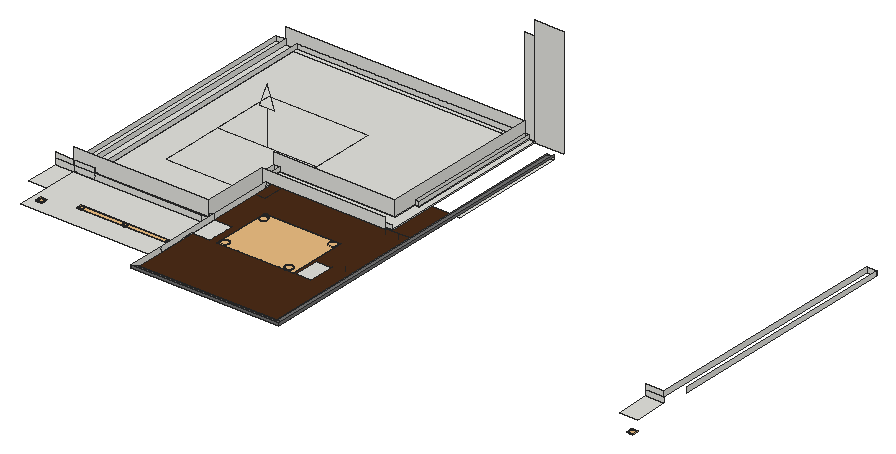
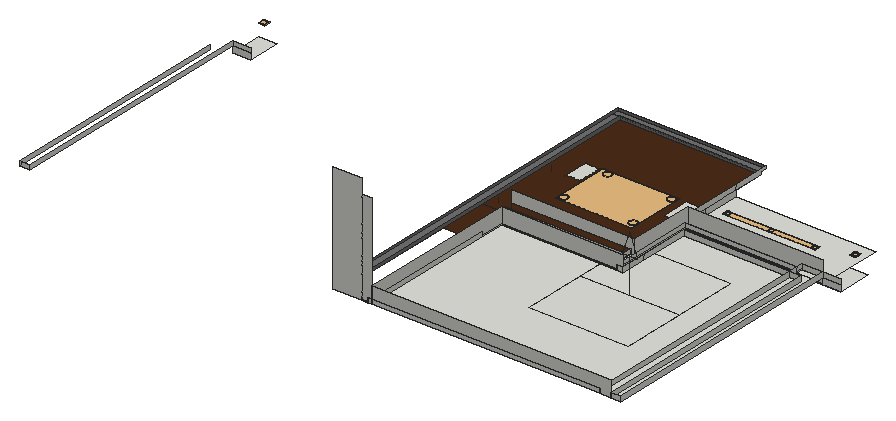
# SketchUp Ruby script. Lengths in inches.
U = 1.inch
M = Sketchup.active_model
def pt(a) = Geom::Point3d.new(a.map { |v| v * U })
def face(e, loops, mat)
  f = e.add_face(loops[0].map { |a| pt(a) })
  loops[1..].each { |l| e.add_face(l.map { |a| pt(a) }).erase! }
  f.material = f.back_material = mat if mat
  f
end
# faces: each face lists its corners as indices into pts; further lists are holes
def faces(e, pts, list, mat = nil) = list.each { |f| face(e, (f[0].is_a?(Array) ? f : [f]).map { |l| l.map { |i| pts[i] } }, mat) }
# xy, xz, yz: faces in a plane at the given z, y or x. An outline is a flat list of corners, or four numbers for a rectangle; further outlines are holes
def ring(l) = l.size == 4 ? [[l[0], l[1]], [l[2], l[1]], [l[2], l[3]], [l[0], l[3]]] : l.each_slice(2).to_a
def flat(e, list, mat, &to3) = list.each { |f| face(e, (f[0].is_a?(Array) ? f : [f]).map { |l| ring(l).map { |u, v| to3.(u, v) } }, mat) }
def xy(e, z, list, mat = nil) = flat(e, list, mat) { |x, y| [x, y, z] }
def xz(e, y, list, mat = nil) = flat(e, list, mat) { |x, z| [x, y, z] }
def yz(e, x, list, mat = nil) = flat(e, list, mat) { |y, z| [x, y, z] }
def lines(e, pts, list) = list.each { |a, b| e.add_line(pt(pts[a]), pt(pts[b])) }
# prism: a flat outline (further loops are holes) pulled along v
def prism(e, loops, v, mat = nil)
  f = face(e, loops, mat); d = Geom::Vector3d.new(v.map { |x| x * U })
  f.pushpull(f.normal.samedirection?(d) ? d.length : -d.length)
end
def box(e, o, s, mat = nil) = prism(e, [[o, [o[0] + s[0], o[1], o[2]], [o[0] + s[0], o[1] + s[1], o[2]], [o[0], o[1] + s[1], o[2]]]], [0, 0, s[2]], mat)
def at(x, y, z, deg = 0) = Geom::Transformation.translation(pt([x, y, z])) * Geom::Transformation.rotation(ORIGIN, Z_AXIS, deg.degrees)
def axes(o, x, y, z) = Geom::Transformation.new([*x, 0, *y, 0, *z, 0, *pt(o).to_a, 1])
def part(name) = M.definitions.add(name)
# library, detail: a bought-in or finely detailed component or shape, given as its bounding box
def library(name, o, s) = part(name).tap { |d| box(d.entities, o, s) }
def detail(e, o, s) = box(e.add_group.entities, o, s)
def put(e, d, t, mat = nil) = e.add_instance(d, t).tap { |i| i.material = mat if mat }
def group(e, t, mat = nil) = e.add_group.tap { |g| g.transformation = t; g.material = mat if mat }.entities
root = M.entities
M.materials.add("[Color M05]").color = [114, 114, 114]
M.materials.add("[Wood Veneer 01]").color = [76, 44, 23]
c1 = library("Group\#26",[-0.5,-0.5,-0.1],[9.125,9.125,0.2])
c2 = library("Group\#20",[-0.5,-0.5,-0.1],[139.5,7.875,0.2])
c3 = library("Group\#21",[-0.5,-0.5,-0.1],[115.36,88.99,0.2])
c4 = part("Group266\#1")
p = [[0,0,0],[0,0,-53.16],[-11.52,0,-53.16],[75.01,-97.09,0],[-75.01,-97.09,0],[75.01,97.09,0],
  [75.01,0,0],[-75.01,97.09,0],[11.52,0,-53.16],[-75.01,0,0],[0,0,-86.05]]
lines(c4.entities,p,[[0,1],[1,2],[3,4],[5,6],[7,5],[1,8],[9,0],[0,6],[8,10],[4,9],[6,3],[2,10],
  [9,7]])
c5 = part("Rectangle Light\#1")
put(c5.entities,c4,at(0,0,0))
xy(root,104.8125,[[252.74,1588.1,279.74,1638.35],[1145.33,1588.1,1172.33,1638.35]])
xy(root,104.9375,[[[279.74,1537.85,491.71,1638.35],[294.3,1555.5,295.35,1555.63,296.33,1556.04,297.18,1556.6875,297.82,1557.53,298.23,1558.51,298.37,1559.56,298.23,1560.61,297.82,1561.59,297.18,1562.43,296.33,1563.08,295.35,1563.48,294.3,1563.62,293.25,1563.48,292.27,1563.08,291.43,1562.43,290.79,1561.59,290.38,1560.61,290.24,1559.56,290.38,1558.51,290.79,1557.53,291.43,1556.6875,292.27,1556.04,293.25,1555.63],[342.36,1572.17,343.25,1572.29,344.08,1572.63,344.79,1573.18,345.34,1573.89,345.68,1574.72,345.8,1575.61,345.68,1576.5,345.34,1577.33,344.79,1578.04,344.08,1578.59,343.25,1578.93,342.36,1579.05,341.47,1578.93,340.64,1578.59,339.93,1578.04,339.38,1577.33,339.04,1576.5,338.92,1575.61,339.04,1574.72,339.38,1573.89,339.93,1573.18,340.64,1572.63,341.47,1572.29],[408.17,1572.17,409.0625,1572.29,409.89,1572.63,410.6,1573.18,411.15,1573.89,411.49,1574.72,411.61,1575.61,411.49,1576.5,411.15,1577.33,410.6,1578.04,409.89,1578.59,409.0625,1578.93,408.17,1579.05,407.28,1578.93,406.45,1578.59,405.74,1578.04,405.2,1577.33,404.85,1576.5,404.74,1575.61,404.85,1574.72,405.2,1573.89,405.74,1573.18,406.45,1572.63,407.28,1572.29],[473.99,1572.17,474.875,1572.29,475.7,1572.63,476.42,1573.18,476.96,1573.89,477.31,1574.72,477.42,1575.61,477.31,1576.5,476.96,1577.33,476.42,1578.04,475.7,1578.59,474.875,1578.93,473.99,1579.05,473.1,1578.93,472.27,1578.59,471.55,1578.04,471.01,1577.33,470.66,1576.5,470.55,1575.61,470.66,1574.72,471.01,1573.89,471.55,1573.18,472.27,1572.63,473.1,1572.29]]])
xy(root,113.8125,[[491.71,1597.35,519.14,1638.29],[649.86,1597.35,671.36,1634.91],[279.74,1638.35,312.05,1647.57],[312.05,1638.35,472.88,1647.57],[279.74,1647.57,312.05,1647.57,312.05,1661.875,294.47,1661.875,294.47,2020.66,279.74,2020.66],
  [294.47,1661.875,312.05,2020.66],[312.05,1661.875,312.05,2013.29,655.66,2013.29,655.66,1775.97,471.68,1775.97,471.68,1661.875],[662.14,1749.22,671.36,2020.66],[704.8,1824.2,715.11,2001.02],[312.05,2013.29,624.8,2020.66],
  [624.8,2013.29,655.66,2020.66]])
xy(root,113.8125,[[[491.71,1490.47,491.71,1597.35,519.14,1597.35,519.14,1638.29,491.71,1638.29,491.71,1749.22,704.8,1749.22,704.8,1490.47],[649.86,1597.35,671.36,1634.91],[633.34,1597.54,634.9,1597.75,636.34,1598.35,637.58,1599.3,638.54,1600.54,639.14,1601.99,639.34,1603.54,639.14,1605.1,638.54,1606.54,637.58,1607.79,636.34,1608.74,634.9,1609.34,633.34,1609.54,631.79,1609.34,630.34,1608.74,629.1,1607.79,628.15,1606.54,627.55,1605.1,627.34,1603.54,627.55,1601.99,628.15,1600.54,629.1,1599.3,630.34,1598.35,631.79,1597.75],[536.53,1597.54,538.08,1597.75,539.53,1598.35,540.77,1599.3,541.73,1600.54,542.33,1601.99,542.53,1603.54,542.33,1605.1,541.73,1606.54,540.77,1607.79,539.53,1608.74,538.08,1609.34,536.53,1609.54,534.98,1609.34,533.53,1608.74,532.29,1607.79,531.33,1606.54,530.73,1605.1,530.53,1603.54,530.73,1601.99,531.33,1600.54,532.29,1599.3,533.53,1598.35,534.98,1597.75],[536.53,1670.29,538.08,1670.5,539.53,1671.1,540.77,1672.05,541.73,1673.29,542.33,1674.74,542.53,1676.29,542.33,1677.85,541.73,1679.29,540.77,1680.54,539.53,1681.49,538.08,1682.09,536.53,1682.29,534.98,1682.09,533.53,1681.49,532.29,1680.54,531.33,1679.29,530.73,1677.85,530.53,1676.29,530.73,1674.74,531.33,1673.29,532.29,1672.05,533.53,1671.1,534.98,1670.5],[638.89,1673.53,640.44,1673.73,641.89,1674.33,643.13,1675.28,644.09,1676.53,644.6875,1677.97,644.89,1679.53,644.6875,1681.08,644.09,1682.53,643.13,1683.77,641.89,1684.72,640.44,1685.32,638.89,1685.53,637.34,1685.32,635.89,1684.72,634.65,1683.77,633.7,1682.53,633.1,1681.08,632.89,1679.53,633.1,1677.97,633.7,1676.53,634.65,1675.28,635.89,1674.33,637.34,1673.73]],[671.36,1749.22,704.8,1824.2]],"[Wood Veneer 01]")
xy(root,115.0625,[[312.05,1638.35,484.3,1638.35,484.3,1737.41,491.71,1737.41,491.71,1749.22,671.36,1749.22,671.36,2020.66,662.14,2020.66,662.14,1813.21,655.66,1813.21,655.66,1775.97,481.36,1775.97,481.36,1647.57,312.05,1647.57]])
xy(root,118.1875,[[491.71,1481.16,715.11,1490.47],[704.8,1490.47,715.11,2001.02]],"[Color M05]")
xz(root,1481.16,[[491.71,118.1875,715.11,121.3125]],"[Color M05]")
xz(root,1490.47,[[491.71,113.8125,704.8,118.1875]],"[Color M05]")
xz(root,1638.35,[[252.74,104.8125,279.74,113.8125],[279.74,104.8125,312.05,104.9375],[1145.33,104.8125,1172.33,113.8125],[279.74,104.9375,312.05,113.8125],[312.05,104.9375,472.88,113.8125],
  [472.88,104.9375,491.71,113.8125],[252.74,113.8125,279.74,121.3125],[279.74,113.8125,312.05,121.3125],[312.05,113.8125,484.3,115.0625],[484.3,113.8125,491.71,121.3125],
  [1145.33,113.8125,1172.33,121.3125],[312.05,115.0625,484.3,115.0625,484.3,138.1875,279.74,138.1875,279.74,121.3125,312.05,121.3125]])
xz(root,1647.57,[[312.05,113.8125,481.36,115.0625],[312.05,115.0625,481.36,121.3125]])
xz(root,1661.875,[[294.47,113.8125,471.68,121.3125]])
xz(root,1737.41,[[484.3,113.8125,491.71,115.0625],[484.3,115.0625,491.71,115.0625,491.71,121.3125,671.36,121.3125,671.36,138.1875,484.3,138.1875]])
xz(root,1749.22,[[491.71,113.8125,662.14,115.0625],[662.14,113.8125,671.36,115.0625],[491.71,115.0625,671.36,121.3125]])
xz(root,1775.97,[[471.68,113.8125,481.36,121.3125],[481.36,113.8125,655.66,115.0625],[481.36,115.0625,655.66,115.0625,655.66,138.1875,471.68,138.1875,471.68,121.3125,481.36,121.3125]])
xz(root,1813.21,[[655.66,113.8125,662.14,115.0625],[655.66,115.0625,662.14,121.3125]])
xz(root,2001.02,[[704.8,113.8125,715.11,118.1875]])
xz(root,2020.66,[[279.74,113.8125,294.47,121.3125],[294.47,113.8125,294.47,138.1875,655.66,138.1875,655.66,121.3125,312.05,121.3125,312.05,113.8125],[312.05,113.8125,655.66,121.3125],[655.66,113.8125,662.14,121.3125],[662.14,113.8125,671.36,115.0625],
  [671.36,113.8125,715.11,279.25],[1172.33,113.8125,1187.0625,121.3125],[662.14,115.0625,662.14,121.3125,655.66,121.3125,655.66,258.1875,671.36,258.1875,671.36,115.0625]])
yz(root,279.74,[[1638.35,113.8125,2020.66,121.3125]])
yz(root,294.47,[[1661.875,113.8125,2020.66,121.3125]])
yz(root,312.05,[[1638.35,113.8125,1647.57,115.0625],[1647.57,113.8125,2020.66,121.3125],[1638.35,115.0625,1647.57,121.3125]])
yz(root,471.68,[[1661.875,113.8125,1737.41,121.3125],[1737.41,113.8125,1775.97,121.3125]])
yz(root,481.36,[[1647.57,113.8125,1775.97,115.0625],[1647.57,115.0625,1775.97,121.3125]])
yz(root,484.3,[[1638.35,113.8125,1737.41,115.0625],[1638.35,115.0625,1737.41,138.1875]])
yz(root,491.71,[[1537.85,104.9375,1597.35,113.8125],[1597.35,104.9375,1638.29,113.8125],[1638.29,104.9375,1638.35,113.8125],[1490.47,113.8125,1490.47,118.1875,1481.16,118.1875,1481.16,121.3125,1537.85,121.3125,1537.85,113.8125],[1537.85,113.8125,1638.35,121.3125],
  [1638.35,113.8125,1737.41,121.3125],[1737.41,113.8125,1749.22,115.0625],[1737.41,115.0625,1749.22,121.3125]])
yz(root,655.66,[[1775.97,113.8125,1813.21,115.0625],[1813.21,113.8125,2020.66,121.3125],[1775.97,115.0625,1813.21,115.0625,1813.21,121.3125,2020.66,121.3125,2020.66,138.1875,1775.97,138.1875]])
yz(root,662.14,[[1813.21,113.8125,2020.66,115.0625],[1813.21,115.0625,2020.66,121.3125]])
yz(root,671.36,[[1749.22,113.8125,2020.66,115.0625]])
yz(root,704.8,[[1490.47,113.8125,2001.02,118.1875]],"[Color M05]")
yz(root,715.11,[[1481.16,118.1875,2001.02,121.3125]],"[Color M05]")
yz(root,1172.33,[[1638.35,113.8125,2020.66,121.3125]])
yz(root,1187.0625,[[1661.875,113.8125,2020.66,121.3125]])
p = [[294.3,1555.5,104.9375],[293.25,1555.63,104.9375],[293.25,1555.63,105.875],[294.3,1555.5,105.875],[295.35,1555.63,104.9375],[295.35,1555.63,105.875],
  [1186.89,1555.5,104.9375],[1185.84,1555.63,104.9375],[1185.84,1555.63,105.875],[1186.89,1555.5,105.875],[292.27,1556.04,104.9375],[292.27,1556.04,105.875],
  [296.33,1556.04,104.9375],[296.33,1556.04,105.875],[1184.86,1556.04,104.9375],[1184.86,1556.04,105.875],[291.43,1556.6875,104.9375],[291.43,1556.6875,105.875],
  [297.18,1556.6875,104.9375],[297.18,1556.6875,105.875],[1184.02,1556.6875,104.9375],[1184.02,1556.6875,105.875],[290.79,1557.53,104.9375],[290.79,1557.53,105.875],
  [297.82,1557.53,104.9375],[297.82,1557.53,105.875],[1183.375,1557.53,104.9375],[1183.375,1557.53,105.875],[290.38,1558.51,104.9375],[290.38,1558.51,105.875],
  [298.23,1558.51,104.9375],[298.23,1558.51,105.875],[1182.97,1558.51,104.9375],[1182.97,1558.51,105.875],[290.24,1559.56,104.9375],[290.24,1559.56,105.875],
  [298.37,1559.56,104.9375],[298.37,1559.56,105.875],[1182.83,1559.56,104.9375],[1182.83,1559.56,105.875],[290.38,1560.61,104.9375],[290.38,1560.61,105.875],
  [298.23,1560.61,104.9375],[298.23,1560.61,105.875],[1182.97,1560.61,104.9375],[1182.97,1560.61,105.875],[290.79,1561.59,104.9375],[290.79,1561.59,105.875],
  [297.82,1561.59,104.9375],[297.82,1561.59,105.875],[1183.375,1561.59,104.9375],[1183.375,1561.59,105.875],[291.43,1562.43,104.9375],[291.43,1562.43,105.875],
  [297.18,1562.43,104.9375],[297.18,1562.43,105.875],[1184.02,1562.43,104.9375],[1184.02,1562.43,105.875],[292.27,1563.08,104.9375],[292.27,1563.08,105.875],
  [296.33,1563.08,104.9375],[296.33,1563.08,105.875],[1184.86,1563.08,104.9375],[1184.86,1563.08,105.875],[293.25,1563.48,104.9375],[293.25,1563.48,105.875],
  [295.35,1563.48,104.9375],[295.35,1563.48,105.875],[1185.84,1563.48,104.9375],[1185.84,1563.48,105.875],[294.3,1563.62,104.9375],[294.3,1563.62,105.875],
  [1186.89,1563.62,104.9375],[1186.89,1563.62,105.875],[342.36,1572.17,104.9375],[341.47,1572.29,104.9375],[341.47,1572.29,105.375],[342.36,1572.17,105.375],
  [343.25,1572.29,104.9375],[343.25,1572.29,105.375],[408.17,1572.17,104.9375],[407.28,1572.29,104.9375],[407.28,1572.29,105.375],[408.17,1572.17,105.375],
  [409.0625,1572.29,104.9375],[409.0625,1572.29,105.375],[473.99,1572.17,104.9375],[473.1,1572.29,104.9375],[473.1,1572.29,105.375],[473.99,1572.17,105.375],
  [474.875,1572.29,104.9375],[474.875,1572.29,105.375],[340.64,1572.63,104.9375],[340.64,1572.63,105.375],[344.08,1572.63,104.9375],[344.08,1572.63,105.375],
  [406.45,1572.63,104.9375],[406.45,1572.63,105.375],[409.89,1572.63,104.9375],[409.89,1572.63,105.375],[472.27,1572.63,104.9375],[472.27,1572.63,105.375],
  [475.7,1572.63,104.9375],[475.7,1572.63,105.375],[339.93,1573.18,104.9375],[339.93,1573.18,105.375],[344.79,1573.18,104.9375],[344.79,1573.18,105.375],
  [405.74,1573.18,104.9375],[405.74,1573.18,105.375],[410.6,1573.18,104.9375],[410.6,1573.18,105.375],[471.55,1573.18,104.9375],[471.55,1573.18,105.375],
  [476.42,1573.18,104.9375],[476.42,1573.18,105.375],[339.38,1573.89,104.9375],[339.38,1573.89,105.375],[345.34,1573.89,104.9375],[345.34,1573.89,105.375],
  [405.2,1573.89,104.9375],[405.2,1573.89,105.375],[411.15,1573.89,104.9375],[411.15,1573.89,105.375],[471.01,1573.89,104.9375],[471.01,1573.89,105.375],
  [476.96,1573.89,104.9375],[476.96,1573.89,105.375],[339.04,1574.72,104.9375],[339.04,1574.72,105.375],[345.68,1574.72,104.9375],[345.68,1574.72,105.375],
  [404.85,1574.72,104.9375],[404.85,1574.72,105.375],[411.49,1574.72,104.9375],[411.49,1574.72,105.375],[470.66,1574.72,104.9375],[470.66,1574.72,105.375],
  [477.31,1574.72,104.9375],[477.31,1574.72,105.375],[338.92,1575.61,104.9375],[338.92,1575.61,105.375],[345.8,1575.61,104.9375],[345.8,1575.61,105.375],
  [404.74,1575.61,104.9375],[404.74,1575.61,105.375],[411.61,1575.61,104.9375],[411.61,1575.61,105.375],[470.55,1575.61,104.9375],[470.55,1575.61,105.375],
  [477.42,1575.61,104.9375],[477.42,1575.61,105.375],[339.04,1576.5,104.9375],[339.04,1576.5,105.375],[345.68,1576.5,104.9375],[345.68,1576.5,105.375],
  [404.85,1576.5,104.9375],[404.85,1576.5,105.375],[411.49,1576.5,104.9375],[411.49,1576.5,105.375],[470.66,1576.5,104.9375],[470.66,1576.5,105.375],
  [477.31,1576.5,104.9375],[477.31,1576.5,105.375],[339.38,1577.33,104.9375],[339.38,1577.33,105.375],[345.34,1577.33,104.9375],[345.34,1577.33,105.375],
  [405.2,1577.33,104.9375],[405.2,1577.33,105.375],[411.15,1577.33,104.9375],[411.15,1577.33,105.375],[471.01,1577.33,104.9375],[471.01,1577.33,105.375],
  [476.96,1577.33,104.9375],[476.96,1577.33,105.375],[339.93,1578.04,104.9375],[339.93,1578.04,105.375],[344.79,1578.04,104.9375],[344.79,1578.04,105.375],
  [405.74,1578.04,104.9375],[405.74,1578.04,105.375],[410.6,1578.04,104.9375],[410.6,1578.04,105.375],[471.55,1578.04,104.9375],[471.55,1578.04,105.375],
  [476.42,1578.04,104.9375],[476.42,1578.04,105.375],[340.64,1578.59,104.9375],[340.64,1578.59,105.375],[344.08,1578.59,104.9375],[344.08,1578.59,105.375],
  [406.45,1578.59,104.9375],[406.45,1578.59,105.375],[409.89,1578.59,104.9375],[409.89,1578.59,105.375],[472.27,1578.59,104.9375],[472.27,1578.59,105.375],
  [475.7,1578.59,104.9375],[475.7,1578.59,105.375],[341.47,1578.93,104.9375],[341.47,1578.93,105.375],[343.25,1578.93,104.9375],[343.25,1578.93,105.375],
  [407.28,1578.93,104.9375],[407.28,1578.93,105.375],[409.0625,1578.93,104.9375],[409.0625,1578.93,105.375],[473.1,1578.93,104.9375],[473.1,1578.93,105.375],
  [474.875,1578.93,104.9375],[474.875,1578.93,105.375],[342.36,1579.05,104.9375],[342.36,1579.05,105.375],[408.17,1579.05,104.9375],[408.17,1579.05,105.375],
  [473.99,1579.05,104.9375],[473.99,1579.05,105.375],[536.53,1597.54,113.8125],[534.98,1597.75,113.8125],[534.98,1597.75,114.6875],[536.53,1597.54,114.6875],
  [538.08,1597.75,113.8125],[538.08,1597.75,114.6875],[633.34,1597.54,113.8125],[631.79,1597.75,113.8125],[631.79,1597.75,114.6875],[633.34,1597.54,114.6875],
  [634.9,1597.75,113.8125],[634.9,1597.75,114.6875],[533.53,1598.35,113.8125],[533.53,1598.35,114.6875],[539.53,1598.35,113.8125],[539.53,1598.35,114.6875],
  [630.34,1598.35,113.8125],[630.34,1598.35,114.6875],[636.34,1598.35,113.8125],[636.34,1598.35,114.6875],[532.29,1599.3,113.8125],[532.29,1599.3,114.6875],
  [540.77,1599.3,113.8125],[540.77,1599.3,114.6875],[629.1,1599.3,113.8125],[629.1,1599.3,114.6875],[637.58,1599.3,113.8125],[637.58,1599.3,114.6875],
  [531.33,1600.54,113.8125],[531.33,1600.54,114.6875],[541.73,1600.54,113.8125],[541.73,1600.54,114.6875],[628.15,1600.54,113.8125],[628.15,1600.54,114.6875],
  [638.54,1600.54,113.8125],[638.54,1600.54,114.6875],[530.73,1601.99,113.8125],[530.73,1601.99,114.6875],[542.33,1601.99,113.8125],[542.33,1601.99,114.6875],
  [627.55,1601.99,113.8125],[627.55,1601.99,114.6875],[639.14,1601.99,113.8125],[639.14,1601.99,114.6875],[530.53,1603.54,113.8125],[530.53,1603.54,114.6875],
  [542.53,1603.54,113.8125],[542.53,1603.54,114.6875],[627.34,1603.54,113.8125],[627.34,1603.54,114.6875],[639.34,1603.54,113.8125],[639.34,1603.54,114.6875],
  [530.73,1605.1,113.8125],[530.73,1605.1,114.6875],[542.33,1605.1,113.8125],[542.33,1605.1,114.6875],[627.55,1605.1,113.8125],[627.55,1605.1,114.6875],
  [639.14,1605.1,113.8125],[639.14,1605.1,114.6875],[531.33,1606.54,113.8125],[531.33,1606.54,114.6875],[541.73,1606.54,113.8125],[541.73,1606.54,114.6875],
  [628.15,1606.54,113.8125],[628.15,1606.54,114.6875],[638.54,1606.54,113.8125],[638.54,1606.54,114.6875],[532.29,1607.79,113.8125],[532.29,1607.79,114.6875],
  [540.77,1607.79,113.8125],[540.77,1607.79,114.6875],[629.1,1607.79,113.8125],[629.1,1607.79,114.6875],[637.58,1607.79,113.8125],[637.58,1607.79,114.6875],
  [533.53,1608.74,113.8125],[533.53,1608.74,114.6875],[539.53,1608.74,113.8125],[539.53,1608.74,114.6875],[630.34,1608.74,113.8125],[630.34,1608.74,114.6875],
  [636.34,1608.74,113.8125],[636.34,1608.74,114.6875],[534.98,1609.34,113.8125],[534.98,1609.34,114.6875],[538.08,1609.34,113.8125],[538.08,1609.34,114.6875],
  [631.79,1609.34,113.8125],[631.79,1609.34,114.6875],[634.9,1609.34,113.8125],[634.9,1609.34,114.6875],[536.53,1609.54,113.8125],[536.53,1609.54,114.6875],
  [633.34,1609.54,113.8125],[633.34,1609.54,114.6875],[536.53,1670.29,113.8125],[534.98,1670.5,113.8125],[534.98,1670.5,114.6875],[536.53,1670.29,114.6875],
  [538.08,1670.5,113.8125],[538.08,1670.5,114.6875],[533.53,1671.1,113.8125],[533.53,1671.1,114.6875],[539.53,1671.1,113.8125],[539.53,1671.1,114.6875],
  [532.29,1672.05,113.8125],[532.29,1672.05,114.6875],[540.77,1672.05,113.8125],[540.77,1672.05,114.6875],[531.33,1673.29,113.8125],[531.33,1673.29,114.6875],
  [541.73,1673.29,113.8125],[541.73,1673.29,114.6875],[530.73,1674.74,113.8125],[530.73,1674.74,114.6875],[542.33,1674.74,113.8125],[542.33,1674.74,114.6875],
  [638.89,1673.53,113.8125],[637.34,1673.73,113.8125],[637.34,1673.73,114.6875],[638.89,1673.53,114.6875],[640.44,1673.73,113.8125],[640.44,1673.73,114.6875],
  [635.89,1674.33,113.8125],[635.89,1674.33,114.6875],[641.89,1674.33,113.8125],[641.89,1674.33,114.6875],[634.65,1675.28,113.8125],[634.65,1675.28,114.6875],
  [643.13,1675.28,113.8125],[643.13,1675.28,114.6875],[530.53,1676.29,113.8125],[530.53,1676.29,114.6875],[542.53,1676.29,113.8125],[542.53,1676.29,114.6875],
  [633.7,1676.53,113.8125],[633.7,1676.53,114.6875],[644.09,1676.53,113.8125],[644.09,1676.53,114.6875],[530.73,1677.85,113.8125],[530.73,1677.85,114.6875],
  [542.33,1677.85,113.8125],[542.33,1677.85,114.6875],[633.1,1677.97,113.8125],[633.1,1677.97,114.6875],[644.6875,1677.97,113.8125],[644.6875,1677.97,114.6875],
  [531.33,1679.29,113.8125],[531.33,1679.29,114.6875],[541.73,1679.29,113.8125],[541.73,1679.29,114.6875],[632.89,1679.53,113.8125],[632.89,1679.53,114.6875],
  [644.89,1679.53,113.8125],[644.89,1679.53,114.6875],[532.29,1680.54,113.8125],[532.29,1680.54,114.6875],[540.77,1680.54,113.8125],[540.77,1680.54,114.6875],
  [633.1,1681.08,113.8125],[633.1,1681.08,114.6875],[644.6875,1681.08,113.8125],[644.6875,1681.08,114.6875],[533.53,1681.49,113.8125],[533.53,1681.49,114.6875],
  [539.53,1681.49,113.8125],[539.53,1681.49,114.6875],[633.7,1682.53,113.8125],[633.7,1682.53,114.6875],[644.09,1682.53,113.8125],[644.09,1682.53,114.6875],
  [534.98,1682.09,113.8125],[534.98,1682.09,114.6875],[538.08,1682.09,113.8125],[538.08,1682.09,114.6875],[536.53,1682.29,113.8125],[536.53,1682.29,114.6875],
  [634.65,1683.77,113.8125],[634.65,1683.77,114.6875],[643.13,1683.77,113.8125],[643.13,1683.77,114.6875],[635.89,1684.72,113.8125],[635.89,1684.72,114.6875],
  [641.89,1684.72,113.8125],[641.89,1684.72,114.6875],[637.34,1685.32,113.8125],[637.34,1685.32,114.6875],[640.44,1685.32,113.8125],[640.44,1685.32,114.6875],
  [638.89,1685.53,113.8125],[638.89,1685.53,114.6875],[690.8,1638.35,113.8125],[690.8,1638.35,121.3125],[690.8,1638.29,113.8125],[690.8,1737.41,121.3125],
  [690.8,1737.41,113.8125],[671.36,1737.41,121.3125],[671.36,1737.41,113.8125],[671.36,1638.29,113.8125],[671.36,1634.91,113.8125]]
faces(root,p,[[0,1,2,3],[4,0,3,5],[6,7,8,9],[1,10,11,2],[12,4,5,13],[7,14,15,8],[10,16,17,11],[18,12,13,19],
  [14,20,21,15],[16,22,23,17],[24,18,19,25],[20,26,27,21],[22,28,29,23],[30,24,25,31],[26,32,33,27],[28,34,35,29],
  [36,30,31,37],[32,38,39,33],[34,40,41,35],[42,36,37,43],[38,44,45,39],[40,46,47,41],[48,42,43,49],[44,50,51,45],
  [46,52,53,47],[54,48,49,55],[50,56,57,51],[52,58,59,53],[60,54,55,61],[56,62,63,57],[58,64,65,59],[66,60,61,67],
  [62,68,69,63],[64,70,71,65],[70,66,67,71],[68,72,73,69],[74,75,76,77],[78,74,77,79],[80,81,82,83],[84,80,83,85],
  [86,87,88,89],[90,86,89,91],[75,92,93,76],[94,78,79,95],[81,96,97,82],[98,84,85,99],[87,100,101,88],[102,90,91,103],
  [92,104,105,93],[106,94,95,107],[96,108,109,97],[110,98,99,111],[100,112,113,101],[114,102,103,115],[104,116,117,105],[118,106,107,119],
  [108,120,121,109],[122,110,111,123],[112,124,125,113],[126,114,115,127],[116,128,129,117],[130,118,119,131],[120,132,133,121],[134,122,123,135],
  [124,136,137,125],[138,126,127,139],[128,140,141,129],[142,130,131,143],[132,144,145,133],[146,134,135,147],[136,148,149,137],[150,138,139,151],
  [140,152,153,141],[154,142,143,155],[144,156,157,145],[158,146,147,159],[148,160,161,149],[162,150,151,163],[152,164,165,153],[166,154,155,167],
  [156,168,169,157],[170,158,159,171],[160,172,173,161],[174,162,163,175],[164,176,177,165],[178,166,167,179],[168,180,181,169],[182,170,171,183],
  [172,184,185,173],[186,174,175,187],[176,188,189,177],[190,178,179,191],[180,192,193,181],[194,182,183,195],[184,196,197,185],[198,186,187,199],
  [188,200,201,189],[202,190,191,203],[192,204,205,193],[206,194,195,207],[196,208,209,197],[210,198,199,211],[200,212,213,201],[212,202,203,213],
  [204,214,215,205],[214,206,207,215],[208,216,217,209],[216,210,211,217]])
faces(root,p,[[218,219,220,221],[222,218,221,223],[224,225,226,227],[228,224,227,229],[219,230,231,220],[232,222,223,233],[225,234,235,226],[236,228,229,237],
  [230,238,239,231],[240,232,233,241],[234,242,243,235],[244,236,237,245],[238,246,247,239],[248,240,241,249],[242,250,251,243],[252,244,245,253],
  [246,254,255,247],[256,248,249,257],[250,258,259,251],[260,252,253,261],[254,262,263,255],[264,256,257,265],[258,266,267,259],[268,260,261,269],
  [262,270,271,263],[272,264,265,273],[266,274,275,267],[276,268,269,277],[270,278,279,271],[280,272,273,281],[274,282,283,275],[284,276,277,285],
  [278,286,287,279],[288,280,281,289],[282,290,291,283],[292,284,285,293],[286,294,295,287],[296,288,289,297],[290,298,299,291],[300,292,293,301],
  [294,302,303,295],[304,296,297,305],[298,306,307,299],[308,300,301,309],[302,310,311,303],[310,304,305,311],[306,312,313,307],[312,308,309,313],
  [314,315,316,317],[318,314,317,319],[315,320,321,316],[322,318,319,323],[320,324,325,321],[326,322,323,327],[324,328,329,325],[330,326,327,331],
  [328,332,333,329],[334,330,331,335],[336,337,338,339],[340,336,339,341],[337,342,343,338],[344,340,341,345],[342,346,347,343],[348,344,345,349],
  [332,350,351,333],[352,334,335,353],[346,354,355,347],[356,348,349,357],[350,358,359,351],[360,352,353,361],[354,362,363,355],[364,356,357,365],
  [358,366,367,359],[368,360,361,369],[362,370,371,363],[372,364,365,373],[366,374,375,367],[376,368,369,377],[370,378,379,371],[380,372,373,381],
  [374,382,383,375],[384,376,377,385],[378,386,387,379],[388,380,381,389],[382,390,391,383],[392,384,385,393],[390,394,395,391],[394,392,393,395],
  [386,396,397,387],[398,388,389,399],[396,400,401,397],[402,398,399,403],[400,404,405,401],[406,402,403,407],[404,408,409,405],[408,406,407,409]],"[Wood Veneer 01]")
lines(root,p,[[410,411],[410,412],[413,414],[415,416],[417,418]])
put(root,c1,at(1182.83,1555.5,105.875))
put(root,c1,at(290.24,1555.5,105.875))
put(root,c2,at(338.92,1572.17,105.375))
put(root,c3,at(530.53,1597.54,114.6875))
put(root,c5,axes([431.33,1814.08,113.82],[1,0,0],[0,1,0],[0,0,-1]))
